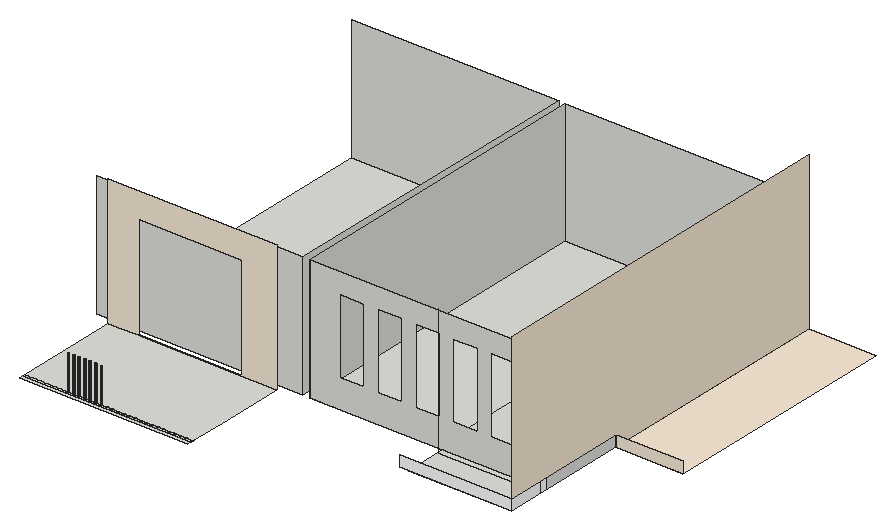
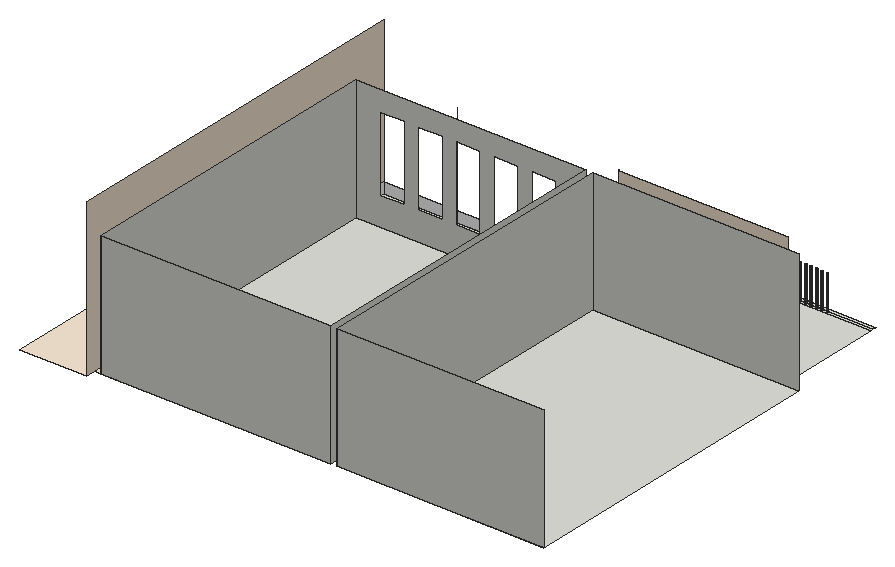
# SketchUp Ruby script. Lengths in inches.
U = 1.inch
M = Sketchup.active_model
def pt(a) = Geom::Point3d.new(a.map { |v| v * U })
def face(e, loops, mat)
  f = e.add_face(loops[0].map { |a| pt(a) })
  loops[1..].each { |l| e.add_face(l.map { |a| pt(a) }).erase! }
  f.material = f.back_material = mat if mat
  f
end
# faces: each face lists its corners as indices into pts; further lists are holes
def faces(e, pts, list, mat = nil) = list.each { |f| face(e, (f[0].is_a?(Array) ? f : [f]).map { |l| l.map { |i| pts[i] } }, mat) }
# xy, xz, yz: faces in a plane at the given z, y or x. An outline is a flat list of corners, or four numbers for a rectangle; further outlines are holes
def ring(l) = l.size == 4 ? [[l[0], l[1]], [l[2], l[1]], [l[2], l[3]], [l[0], l[3]]] : l.each_slice(2).to_a
def flat(e, list, mat, &to3) = list.each { |f| face(e, (f[0].is_a?(Array) ? f : [f]).map { |l| ring(l).map { |u, v| to3.(u, v) } }, mat) }
def xy(e, z, list, mat = nil) = flat(e, list, mat) { |x, y| [x, y, z] }
def xz(e, y, list, mat = nil) = flat(e, list, mat) { |x, z| [x, y, z] }
def yz(e, x, list, mat = nil) = flat(e, list, mat) { |y, z| [x, y, z] }
def lines(e, pts, list) = list.each { |a, b| e.add_line(pt(pts[a]), pt(pts[b])) }
# prism: a flat outline (further loops are holes) pulled along v
def prism(e, loops, v, mat = nil)
  f = face(e, loops, mat); d = Geom::Vector3d.new(v.map { |x| x * U })
  f.pushpull(f.normal.samedirection?(d) ? d.length : -d.length)
end
def box(e, o, s, mat = nil) = prism(e, [[o, [o[0] + s[0], o[1], o[2]], [o[0] + s[0], o[1] + s[1], o[2]], [o[0], o[1] + s[1], o[2]]]], [0, 0, s[2]], mat)
def at(x, y, z, deg = 0) = Geom::Transformation.translation(pt([x, y, z])) * Geom::Transformation.rotation(ORIGIN, Z_AXIS, deg.degrees)
def axes(o, x, y, z) = Geom::Transformation.new([*x, 0, *y, 0, *z, 0, *pt(o).to_a, 1])
def part(name) = M.definitions.add(name)
# library, detail: a bought-in or finely detailed component or shape, given as its bounding box
def library(name, o, s) = part(name).tap { |d| box(d.entities, o, s) }
def detail(e, o, s) = box(e.add_group.entities, o, s)
def put(e, d, t, mat = nil) = e.add_instance(d, t).tap { |i| i.material = mat if mat }
def group(e, t, mat = nil) = e.add_group.tap { |g| g.transformation = t; g.material = mat if mat }.entities
root = M.entities
M.materials.add("[0028_AntiqueWhite]").color = [250, 235, 215]
M.materials.add("[Color M00]").color = [255, 255, 255]
M.materials.add("[Color M08]").color = [30, 30, 30]
xy(root,321,[[206.51,190.32,206.52,193.51,50.75,193.51,50.75,190.5],[206.52,193.51,206.5625,231.9375,206.63,292.44,206.5625,292.44,177.59,292.48,76.05,292.6,50.75,292.625,50.68,231.9375,50.75,231.9375,50.75,196.625,206.52,196.625],[[50.75,193.51,206.52,196.625],[55.99,194.51,55.8,194.57,55.63,194.67,55.5,194.81,55.41,194.99,55.36,195.18,55.37,195.375,55.42,195.5625,55.53,195.73,55.67,195.86,55.84,195.95,56.03,196,56.23,195.99,56.42,195.9375,56.58,195.83,56.72,195.69,56.81,195.52,56.85,195.33,56.85,195.13,56.79,194.95,56.6875,194.78,56.55,194.64,56.375,194.55,56.18,194.51],[61.05,194.51,60.86,194.57,60.7,194.67,60.5625,194.81,60.47,194.99,60.42,195.18,60.43,195.375,60.49,195.5625,60.59,195.73,60.73,195.86,60.9,195.95,61.1,196,61.29,195.99,61.48,195.9375,61.65,195.83,61.78,195.69,61.87,195.52,61.92,195.33,61.91,195.13,61.85,194.95,61.75,194.78,61.61,194.64,61.4375,194.55,61.25,194.51],[66.11,194.51,65.93,194.57,65.76,194.67,65.625,194.81,65.53,194.99,65.49,195.18,65.49,195.375,65.55,195.5625,65.65,195.73,65.79,195.86,65.97,195.95,66.16,196,66.35,195.99,66.54,195.9375,66.71,195.83,66.84,195.69,66.93,195.52,66.98,195.33,66.97,195.13,66.92,194.95,66.8125,194.78,66.67,194.64,66.5,194.55,66.31,194.51],[71.18,194.51,70.99,194.57,70.82,194.67,70.6875,194.81,70.59,194.99,70.55,195.18,70.56,195.375,70.61,195.5625,70.71,195.73,70.86,195.86,71.03,195.95,71.22,196,71.42,195.99,71.6,195.9375,71.77,195.83,71.9,195.69,72,195.52,72.04,195.33,72.04,195.13,71.98,194.95,71.875,194.78,71.73,194.64,71.5625,194.55,71.37,194.51],[76.24,194.51,76.05,194.57,75.88,194.67,75.75,194.81,75.66,194.99,75.61,195.18,75.62,195.375,75.67,195.5625,75.78,195.73,75.92,195.86,76.09,195.95,76.28,196,76.48,195.99,76.67,195.9375,76.83,195.83,76.97,195.69,77.06,195.52,77.1,195.33,77.1,195.13,77.04,194.95,76.9375,194.78,76.8,194.64,76.625,194.55,76.43,194.51],[81.3,194.51,81.11,194.57,80.95,194.67,80.8125,194.81,80.72,194.99,80.67,195.18,80.68,195.375,80.74,195.5625,80.84,195.73,80.98,195.86,81.15,195.95,81.35,196,81.54,195.99,81.73,195.9375,81.9,195.83,82.03,195.69,82.12,195.52,82.17,195.33,82.16,195.13,82.1,194.95,82,194.78,81.86,194.64,81.6875,194.55,81.5,194.51],[86.36,194.51,86.18,194.57,86.01,194.67,85.875,194.81,85.78,194.99,85.74,195.18,85.74,195.375,85.8,195.5625,85.9,195.73,86.04,195.86,86.22,195.95,86.41,196,86.6,195.99,86.79,195.9375,86.96,195.83,87.09,195.69,87.18,195.52,87.23,195.33,87.22,195.13,87.17,194.95,87.0625,194.78,86.92,194.64,86.75,194.55,86.56,194.51],[91.43,194.51,91.24,194.57,91.07,194.67,90.9375,194.81,90.84,194.99,90.8,195.18,90.81,195.375,90.86,195.5625,90.96,195.73,91.11,195.86,91.28,195.95,91.47,196,91.67,195.99,91.85,195.9375,92.02,195.83,92.15,195.69,92.25,195.52,92.29,195.33,92.29,195.13,92.23,194.95,92.125,194.78,91.98,194.64,91.8125,194.55,91.62,194.51],[96.49,194.51,96.3,194.57,96.13,194.67,96,194.81,95.91,194.99,95.86,195.18,95.87,195.375,95.92,195.5625,96.03,195.73,96.17,195.86,96.34,195.95,96.53,196,96.73,195.99,96.92,195.9375,97.08,195.83,97.22,195.69,97.31,195.52,97.35,195.33,97.35,195.13,97.29,194.95,97.1875,194.78,97.05,194.64,96.875,194.55,96.68,194.51],[101.55,194.51,101.36,194.57,101.2,194.67,101.0625,194.81,100.97,194.99,100.92,195.18,100.93,195.375,100.99,195.5625,101.09,195.73,101.23,195.86,101.4,195.95,101.6,196,101.79,195.99,101.98,195.9375,102.15,195.83,102.28,195.69,102.37,195.52,102.42,195.33,102.41,195.13,102.35,194.95,102.25,194.78,102.11,194.64,101.9375,194.55,101.75,194.51],[106.61,194.51,106.43,194.57,106.26,194.67,106.125,194.81,106.03,194.99,105.99,195.18,105.99,195.375,106.05,195.5625,106.15,195.73,106.29,195.86,106.47,195.95,106.66,196,106.85,195.99,107.04,195.9375,107.21,195.83,107.34,195.69,107.43,195.52,107.48,195.33,107.47,195.13,107.42,194.95,107.3125,194.78,107.17,194.64,107,194.55,106.81,194.51],[111.68,194.51,111.49,194.57,111.32,194.67,111.1875,194.81,111.09,194.99,111.05,195.18,111.06,195.375,111.11,195.5625,111.21,195.73,111.36,195.86,111.53,195.95,111.72,196,111.92,195.99,112.1,195.9375,112.27,195.83,112.4,195.69,112.5,195.52,112.54,195.33,112.54,195.13,112.48,194.95,112.375,194.78,112.23,194.64,112.0625,194.55,111.87,194.51],[116.74,194.51,116.55,194.57,116.38,194.67,116.25,194.81,116.16,194.99,116.11,195.18,116.12,195.375,116.17,195.5625,116.28,195.73,116.42,195.86,116.59,195.95,116.78,196,116.98,195.99,117.17,195.9375,117.33,195.83,117.47,195.69,117.56,195.52,117.6,195.33,117.6,195.13,117.54,194.95,117.4375,194.78,117.3,194.64,117.125,194.55,116.93,194.51],[121.8,194.51,121.61,194.57,121.45,194.67,121.3125,194.81,121.22,194.99,121.17,195.18,121.18,195.375,121.24,195.5625,121.34,195.73,121.48,195.86,121.65,195.95,121.85,196,122.04,195.99,122.23,195.9375,122.4,195.83,122.53,195.69,122.62,195.52,122.67,195.33,122.66,195.13,122.6,194.95,122.5,194.78,122.36,194.64,122.1875,194.55,122,194.51],[126.86,194.51,126.68,194.57,126.51,194.67,126.375,194.81,126.28,194.99,126.24,195.18,126.24,195.375,126.3,195.5625,126.4,195.73,126.54,195.86,126.72,195.95,126.91,196,127.1,195.99,127.29,195.9375,127.46,195.83,127.59,195.69,127.68,195.52,127.73,195.33,127.72,195.13,127.67,194.95,127.5625,194.78,127.42,194.64,127.25,194.55,127.06,194.51],[132.11,194.51,131.93,194.57,131.76,194.67,131.625,194.81,131.53,194.99,131.49,195.18,131.49,195.375,131.55,195.5625,131.65,195.73,131.79,195.86,131.97,195.95,132.16,196,132.35,195.99,132.54,195.9375,132.71,195.83,132.84,195.69,132.93,195.52,132.98,195.33,132.97,195.13,132.92,194.95,132.8125,194.78,132.67,194.64,132.5,194.55,132.31,194.51],[137.36,194.51,137.18,194.57,137.01,194.67,136.875,194.81,136.78,194.99,136.74,195.18,136.74,195.375,136.8,195.5625,136.9,195.73,137.04,195.86,137.22,195.95,137.41,196,137.6,195.99,137.79,195.9375,137.96,195.83,138.09,195.69,138.18,195.52,138.23,195.33,138.22,195.13,138.17,194.95,138.0625,194.78,137.92,194.64,137.75,194.55,137.56,194.51],[142.61,194.51,142.43,194.57,142.26,194.67,142.125,194.81,142.03,194.99,141.99,195.18,141.99,195.375,142.05,195.5625,142.15,195.73,142.29,195.86,142.47,195.95,142.66,196,142.85,195.99,143.04,195.9375,143.21,195.83,143.34,195.69,143.43,195.52,143.48,195.33,143.47,195.13,143.42,194.95,143.3125,194.78,143.17,194.64,143,194.55,142.81,194.51],[147.86,194.51,147.68,194.57,147.51,194.67,147.375,194.81,147.28,194.99,147.24,195.18,147.24,195.375,147.3,195.5625,147.4,195.73,147.54,195.86,147.72,195.95,147.91,196,148.1,195.99,148.29,195.9375,148.46,195.83,148.59,195.69,148.68,195.52,148.73,195.33,148.72,195.13,148.67,194.95,148.5625,194.78,148.42,194.64,148.25,194.55,148.06,194.51],[153.11,194.51,152.93,194.57,152.76,194.67,152.625,194.81,152.53,194.99,152.49,195.18,152.49,195.375,152.55,195.5625,152.65,195.73,152.79,195.86,152.97,195.95,153.16,196,153.35,195.99,153.54,195.9375,153.71,195.83,153.84,195.69,153.93,195.52,153.98,195.33,153.97,195.13,153.92,194.95,153.8125,194.78,153.67,194.64,153.5,194.55,153.31,194.51],[158.36,194.51,158.18,194.57,158.01,194.67,157.875,194.81,157.78,194.99,157.74,195.18,157.74,195.375,157.8,195.5625,157.9,195.73,158.04,195.86,158.22,195.95,158.41,196,158.6,195.99,158.79,195.9375,158.96,195.83,159.09,195.69,159.18,195.52,159.23,195.33,159.22,195.13,159.17,194.95,159.0625,194.78,158.92,194.64,158.75,194.55,158.56,194.51],[163.61,194.51,163.43,194.57,163.26,194.67,163.125,194.81,163.03,194.99,162.99,195.18,162.99,195.375,163.05,195.5625,163.15,195.73,163.29,195.86,163.47,195.95,163.66,196,163.85,195.99,164.04,195.9375,164.21,195.83,164.34,195.69,164.43,195.52,164.48,195.33,164.47,195.13,164.42,194.95,164.3125,194.78,164.17,194.64,164,194.55,163.81,194.51],[168.86,194.51,168.68,194.57,168.51,194.67,168.375,194.81,168.28,194.99,168.24,195.18,168.24,195.375,168.3,195.5625,168.4,195.73,168.54,195.86,168.72,195.95,168.91,196,169.1,195.99,169.29,195.9375,169.46,195.83,169.59,195.69,169.68,195.52,169.73,195.33,169.72,195.13,169.67,194.95,169.5625,194.78,169.42,194.64,169.25,194.55,169.06,194.51],[174.11,194.51,173.93,194.57,173.76,194.67,173.625,194.81,173.53,194.99,173.49,195.18,173.49,195.375,173.55,195.5625,173.65,195.73,173.79,195.86,173.97,195.95,174.16,196,174.35,195.99,174.54,195.9375,174.71,195.83,174.84,195.69,174.93,195.52,174.98,195.33,174.97,195.13,174.92,194.95,174.8125,194.78,174.67,194.64,174.5,194.55,174.31,194.51],[179.36,194.51,179.18,194.57,179.01,194.67,178.875,194.81,178.78,194.99,178.74,195.18,178.74,195.375,178.8,195.5625,178.9,195.73,179.04,195.86,179.22,195.95,179.41,196,179.6,195.99,179.79,195.9375,179.96,195.83,180.09,195.69,180.18,195.52,180.23,195.33,180.22,195.13,180.17,194.95,180.0625,194.78,179.92,194.64,179.75,194.55,179.56,194.51],[184.61,194.51,184.43,194.57,184.26,194.67,184.125,194.81,184.03,194.99,183.99,195.18,183.99,195.375,184.05,195.5625,184.15,195.73,184.29,195.86,184.47,195.95,184.66,196,184.85,195.99,185.04,195.9375,185.21,195.83,185.34,195.69,185.43,195.52,185.48,195.33,185.47,195.13,185.42,194.95,185.3125,194.78,185.17,194.64,185,194.55,184.81,194.51],[189.86,194.51,189.68,194.57,189.51,194.67,189.375,194.81,189.28,194.99,189.24,195.18,189.24,195.375,189.3,195.5625,189.4,195.73,189.54,195.86,189.72,195.95,189.91,196,190.1,195.99,190.29,195.9375,190.46,195.83,190.59,195.69,190.68,195.52,190.73,195.33,190.72,195.13,190.67,194.95,190.5625,194.78,190.42,194.64,190.25,194.55,190.06,194.51],[195.11,194.51,194.93,194.57,194.76,194.67,194.625,194.81,194.53,194.99,194.49,195.18,194.49,195.375,194.55,195.5625,194.65,195.73,194.79,195.86,194.97,195.95,195.16,196,195.35,195.99,195.54,195.9375,195.71,195.83,195.84,195.69,195.93,195.52,195.98,195.33,195.97,195.13,195.92,194.95,195.8125,194.78,195.67,194.64,195.5,194.55,195.31,194.51],[200.36,194.51,200.18,194.57,200.01,194.67,199.875,194.81,199.78,194.99,199.74,195.18,199.74,195.375,199.8,195.5625,199.9,195.73,200.04,195.86,200.22,195.95,200.41,196,200.6,195.99,200.79,195.9375,200.96,195.83,201.09,195.69,201.18,195.52,201.23,195.33,201.22,195.13,201.17,194.95,201.0625,194.78,200.92,194.64,200.75,194.55,200.56,194.51],[205.61,194.51,205.43,194.57,205.26,194.67,205.125,194.81,205.03,194.99,204.99,195.18,204.99,195.375,205.05,195.5625,205.15,195.73,205.29,195.86,205.47,195.95,205.66,196,205.85,195.99,206.04,195.9375,206.21,195.83,206.34,195.69,206.43,195.52,206.48,195.33,206.47,195.13,206.42,194.95,206.3125,194.78,206.17,194.64,206,194.55,205.81,194.51]],[355.625,259.125,450.25,292.4375],[355.625,292.4375,450.25,298.4375],
  [35.1875,298.4375,226.3125,592.9375],[232.3125,298.4375,349.625,592.9375],[349.625,298.4375,444.4375,592.9375],[444.4375,298.4375,450.25,379.25],[444.4375,379.25,450.25,384.87]])
xy(root,321,[[450.25,379.25,512.4375,601.9375],[444.4375,384.87,450.25,592.9375]],"[0028_AntiqueWhite]")
xy(root,321,[[91.43,194.51,91.24,194.57,91.07,194.67,90.9375,194.81,90.84,194.99,90.8,195.18,90.81,195.375,90.86,195.5625,90.96,195.73,91.11,195.86,91.28,195.95,91.47,196,91.67,195.99,91.85,195.9375,92.02,195.83,92.15,195.69,92.25,195.52,92.29,195.33,92.29,195.13,92.23,194.95,92.125,194.78,91.98,194.64,91.8125,194.55,91.62,194.51],[96.49,194.51,96.3,194.57,96.13,194.67,96,194.81,95.91,194.99,95.86,195.18,95.87,195.375,95.92,195.5625,96.03,195.73,96.17,195.86,96.34,195.95,96.53,196,96.73,195.99,96.92,195.9375,97.08,195.83,97.22,195.69,97.31,195.52,97.35,195.33,97.35,195.13,97.29,194.95,97.1875,194.78,97.05,194.64,96.875,194.55,96.68,194.51],[101.55,194.51,101.36,194.57,101.2,194.67,101.0625,194.81,100.97,194.99,100.92,195.18,100.93,195.375,100.99,195.5625,101.09,195.73,101.23,195.86,101.4,195.95,101.6,196,101.79,195.99,101.98,195.9375,102.15,195.83,102.28,195.69,102.37,195.52,102.42,195.33,102.41,195.13,102.35,194.95,102.25,194.78,102.11,194.64,101.9375,194.55,101.75,194.51],[106.61,194.51,106.43,194.57,106.26,194.67,106.125,194.81,106.03,194.99,105.99,195.18,105.99,195.375,106.05,195.5625,106.15,195.73,106.29,195.86,106.47,195.95,106.66,196,106.85,195.99,107.04,195.9375,107.21,195.83,107.34,195.69,107.43,195.52,107.48,195.33,107.47,195.13,107.42,194.95,107.3125,194.78,107.17,194.64,107,194.55,106.81,194.51],[111.68,194.51,111.49,194.57,111.32,194.67,111.1875,194.81,111.09,194.99,111.05,195.18,111.06,195.375,111.11,195.5625,111.21,195.73,111.36,195.86,111.53,195.95,111.72,196,111.92,195.99,112.1,195.9375,112.27,195.83,112.4,195.69,112.5,195.52,112.54,195.33,112.54,195.13,112.48,194.95,112.375,194.78,112.23,194.64,112.0625,194.55,111.87,194.51],
  [116.74,194.51,116.55,194.57,116.38,194.67,116.25,194.81,116.16,194.99,116.11,195.18,116.12,195.375,116.17,195.5625,116.28,195.73,116.42,195.86,116.59,195.95,116.78,196,116.98,195.99,117.17,195.9375,117.33,195.83,117.47,195.69,117.56,195.52,117.6,195.33,117.6,195.13,117.54,194.95,117.4375,194.78,117.3,194.64,117.125,194.55,116.93,194.51],[121.8,194.51,121.61,194.57,121.45,194.67,121.3125,194.81,121.22,194.99,121.17,195.18,121.18,195.375,121.24,195.5625,121.34,195.73,121.48,195.86,121.65,195.95,121.85,196,122.04,195.99,122.23,195.9375,122.4,195.83,122.53,195.69,122.62,195.52,122.67,195.33,122.66,195.13,122.6,194.95,122.5,194.78,122.36,194.64,122.1875,194.55,122,194.51],[126.86,194.51,126.68,194.57,126.51,194.67,126.375,194.81,126.28,194.99,126.24,195.18,126.24,195.375,126.3,195.5625,126.4,195.73,126.54,195.86,126.72,195.95,126.91,196,127.1,195.99,127.29,195.9375,127.46,195.83,127.59,195.69,127.68,195.52,127.73,195.33,127.72,195.13,127.67,194.95,127.5625,194.78,127.42,194.64,127.25,194.55,127.06,194.51],[132.11,194.51,131.93,194.57,131.76,194.67,131.625,194.81,131.53,194.99,131.49,195.18,131.49,195.375,131.55,195.5625,131.65,195.73,131.79,195.86,131.97,195.95,132.16,196,132.35,195.99,132.54,195.9375,132.71,195.83,132.84,195.69,132.93,195.52,132.98,195.33,132.97,195.13,132.92,194.95,132.8125,194.78,132.67,194.64,132.5,194.55,132.31,194.51],[137.36,194.51,137.18,194.57,137.01,194.67,136.875,194.81,136.78,194.99,136.74,195.18,136.74,195.375,136.8,195.5625,136.9,195.73,137.04,195.86,137.22,195.95,137.41,196,137.6,195.99,137.79,195.9375,137.96,195.83,138.09,195.69,138.18,195.52,138.23,195.33,138.22,195.13,138.17,194.95,138.0625,194.78,137.92,194.64,137.75,194.55,137.56,194.51],
  [142.61,194.51,142.43,194.57,142.26,194.67,142.125,194.81,142.03,194.99,141.99,195.18,141.99,195.375,142.05,195.5625,142.15,195.73,142.29,195.86,142.47,195.95,142.66,196,142.85,195.99,143.04,195.9375,143.21,195.83,143.34,195.69,143.43,195.52,143.48,195.33,143.47,195.13,143.42,194.95,143.3125,194.78,143.17,194.64,143,194.55,142.81,194.51],[147.86,194.51,147.68,194.57,147.51,194.67,147.375,194.81,147.28,194.99,147.24,195.18,147.24,195.375,147.3,195.5625,147.4,195.73,147.54,195.86,147.72,195.95,147.91,196,148.1,195.99,148.29,195.9375,148.46,195.83,148.59,195.69,148.68,195.52,148.73,195.33,148.72,195.13,148.67,194.95,148.5625,194.78,148.42,194.64,148.25,194.55,148.06,194.51],[153.11,194.51,152.93,194.57,152.76,194.67,152.625,194.81,152.53,194.99,152.49,195.18,152.49,195.375,152.55,195.5625,152.65,195.73,152.79,195.86,152.97,195.95,153.16,196,153.35,195.99,153.54,195.9375,153.71,195.83,153.84,195.69,153.93,195.52,153.98,195.33,153.97,195.13,153.92,194.95,153.8125,194.78,153.67,194.64,153.5,194.55,153.31,194.51],[158.36,194.51,158.18,194.57,158.01,194.67,157.875,194.81,157.78,194.99,157.74,195.18,157.74,195.375,157.8,195.5625,157.9,195.73,158.04,195.86,158.22,195.95,158.41,196,158.6,195.99,158.79,195.9375,158.96,195.83,159.09,195.69,159.18,195.52,159.23,195.33,159.22,195.13,159.17,194.95,159.0625,194.78,158.92,194.64,158.75,194.55,158.56,194.51],[163.61,194.51,163.43,194.57,163.26,194.67,163.125,194.81,163.03,194.99,162.99,195.18,162.99,195.375,163.05,195.5625,163.15,195.73,163.29,195.86,163.47,195.95,163.66,196,163.85,195.99,164.04,195.9375,164.21,195.83,164.34,195.69,164.43,195.52,164.48,195.33,164.47,195.13,164.42,194.95,164.3125,194.78,164.17,194.64,164,194.55,163.81,194.51],
  [168.86,194.51,168.68,194.57,168.51,194.67,168.375,194.81,168.28,194.99,168.24,195.18,168.24,195.375,168.3,195.5625,168.4,195.73,168.54,195.86,168.72,195.95,168.91,196,169.1,195.99,169.29,195.9375,169.46,195.83,169.59,195.69,169.68,195.52,169.73,195.33,169.72,195.13,169.67,194.95,169.5625,194.78,169.42,194.64,169.25,194.55,169.06,194.51],[174.11,194.51,173.93,194.57,173.76,194.67,173.625,194.81,173.53,194.99,173.49,195.18,173.49,195.375,173.55,195.5625,173.65,195.73,173.79,195.86,173.97,195.95,174.16,196,174.35,195.99,174.54,195.9375,174.71,195.83,174.84,195.69,174.93,195.52,174.98,195.33,174.97,195.13,174.92,194.95,174.8125,194.78,174.67,194.64,174.5,194.55,174.31,194.51],[179.36,194.51,179.18,194.57,179.01,194.67,178.875,194.81,178.78,194.99,178.74,195.18,178.74,195.375,178.8,195.5625,178.9,195.73,179.04,195.86,179.22,195.95,179.41,196,179.6,195.99,179.79,195.9375,179.96,195.83,180.09,195.69,180.18,195.52,180.23,195.33,180.22,195.13,180.17,194.95,180.0625,194.78,179.92,194.64,179.75,194.55,179.56,194.51],[184.61,194.51,184.43,194.57,184.26,194.67,184.125,194.81,184.03,194.99,183.99,195.18,183.99,195.375,184.05,195.5625,184.15,195.73,184.29,195.86,184.47,195.95,184.66,196,184.85,195.99,185.04,195.9375,185.21,195.83,185.34,195.69,185.43,195.52,185.48,195.33,185.47,195.13,185.42,194.95,185.3125,194.78,185.17,194.64,185,194.55,184.81,194.51],[189.86,194.51,189.68,194.57,189.51,194.67,189.375,194.81,189.28,194.99,189.24,195.18,189.24,195.375,189.3,195.5625,189.4,195.73,189.54,195.86,189.72,195.95,189.91,196,190.1,195.99,190.29,195.9375,190.46,195.83,190.59,195.69,190.68,195.52,190.73,195.33,190.72,195.13,190.67,194.95,190.5625,194.78,190.42,194.64,190.25,194.55,190.06,194.51],
  [195.11,194.51,194.93,194.57,194.76,194.67,194.625,194.81,194.53,194.99,194.49,195.18,194.49,195.375,194.55,195.5625,194.65,195.73,194.79,195.86,194.97,195.95,195.16,196,195.35,195.99,195.54,195.9375,195.71,195.83,195.84,195.69,195.93,195.52,195.98,195.33,195.97,195.13,195.92,194.95,195.8125,194.78,195.67,194.64,195.5,194.55,195.31,194.51],[200.36,194.51,200.18,194.57,200.01,194.67,199.875,194.81,199.78,194.99,199.74,195.18,199.74,195.375,199.8,195.5625,199.9,195.73,200.04,195.86,200.22,195.95,200.41,196,200.6,195.99,200.79,195.9375,200.96,195.83,201.09,195.69,201.18,195.52,201.23,195.33,201.22,195.13,201.17,194.95,201.0625,194.78,200.92,194.64,200.75,194.55,200.56,194.51],[205.61,194.51,205.43,194.57,205.26,194.67,205.125,194.81,205.03,194.99,204.99,195.18,204.99,195.375,205.05,195.5625,205.15,195.73,205.29,195.86,205.47,195.95,205.66,196,205.85,195.99,206.04,195.9375,206.21,195.83,206.34,195.69,206.43,195.52,206.48,195.33,206.47,195.13,206.42,194.95,206.3125,194.78,206.17,194.64,206,194.55,205.81,194.51]],"[Color M08]")
xz(root,194.51,[[91.43,321,91.62,353.72],[96.49,321,96.68,353.72],[101.55,321,101.75,353.72],[106.61,321,106.81,353.72],[111.68,321,111.87,353.72],
  [116.74,321,116.93,353.72]],"[Color M08]")
xz(root,259.125,[[346.5625,321,450.25,331.3125]],"[Color M00]")
xz(root,298.4375,[[35.1875,321,226.3125,435],[[232.3125,321,444.4375,435],[329.81,347.02,352.43,416.46],[364.87,347.02,387.5,416.46],[399.93,347.02,422.56,416.46],[294.75,347.02,317.37,416.46],[259.68,347.02,282.31,416.46]]])
xz(root,379.25,[[450.25,321,512.4375,331.3125]],"[0028_AntiqueWhite]")
xz(root,592.9375,[[35.1875,321,226.3125,435],[232.3125,321,444.4375,435]])
yz(root,92.29,[[195.13,321,195.33,353.72]],"[Color M08]")
yz(root,97.35,[[195.13,321,195.33,353.72]],"[Color M08]")
yz(root,105.99,[[195.18,321,195.375,353.72]],"[Color M08]")
yz(root,112.54,[[195.13,321,195.33,353.72]],"[Color M08]")
yz(root,117.6,[[195.13,321,195.33,353.72]],"[Color M08]")
yz(root,226.3125,[[298.4375,321,592.9375,435]])
yz(root,232.3125,[[298.4375,321,592.9375,435]])
yz(root,444.4375,[[298.4375,321,592.9375,435]])
yz(root,450.25,[[298.4375,321,379.25,331.3125]])
yz(root,450.25,[[379.25,321,601.9375,321,601.9375,465,259.125,465,259.125,331.3125,379.25,331.3125]],"[0028_AntiqueWhite]")
yz(root,450.25,[[259.125,321,292.4375,331.3125],[292.4375,321,298.4375,331.3125]],"[Color M00]")
p = [[91.62,194.51,321],[91.8125,194.55,321],[91.8125,194.55,353.72],[91.62,194.51,353.72],[96.3,194.57,321],[96.49,194.51,321],
  [96.49,194.51,353.72],[96.3,194.57,353.72],[96.68,194.51,321],[96.875,194.55,321],[96.875,194.55,353.72],[96.68,194.51,353.72],
  [101.36,194.57,321],[101.55,194.51,321],[101.55,194.51,353.72],[101.36,194.57,353.72],[101.75,194.51,321],[101.9375,194.55,321],
  [101.9375,194.55,353.72],[101.75,194.51,353.72],[106.43,194.57,321],[106.61,194.51,321],[106.61,194.51,353.72],[106.43,194.57,353.72],
  [106.81,194.51,321],[107,194.55,321],[107,194.55,353.72],[106.81,194.51,353.72],[111.49,194.57,321],[111.68,194.51,321],
  [111.68,194.51,353.72],[111.49,194.57,353.72],[111.87,194.51,321],[112.0625,194.55,321],[112.0625,194.55,353.72],[111.87,194.51,353.72],
  [116.55,194.57,321],[116.74,194.51,321],[116.74,194.51,353.72],[116.55,194.57,353.72],[116.93,194.51,321],[117.125,194.55,321],
  [117.125,194.55,353.72],[116.93,194.51,353.72],[91.98,194.64,321],[91.98,194.64,353.72],[92.125,194.78,321],[92.125,194.78,353.72],
  [96.13,194.67,321],[96.13,194.67,353.72],[97.05,194.64,321],[97.05,194.64,353.72],[97.1875,194.78,321],[97.1875,194.78,353.72],
  [101.2,194.67,321],[101.2,194.67,353.72],[102.11,194.64,321],[102.11,194.64,353.72],[102.25,194.78,321],[102.25,194.78,353.72],
  [106.26,194.67,321],[106.26,194.67,353.72],[107.17,194.64,321],[107.17,194.64,353.72],[107.3125,194.78,321],[107.3125,194.78,353.72],
  [111.32,194.67,321],[111.32,194.67,353.72],[112.23,194.64,321],[112.23,194.64,353.72],[112.375,194.78,321],[112.375,194.78,353.72],
  [116.38,194.67,321],[116.38,194.67,353.72],[117.3,194.64,321],[117.3,194.64,353.72],[117.4375,194.78,321],[117.4375,194.78,353.72],
  [122.36,194.64,321],[122.5,194.78,321],[122.5,194.78,353.72],[122.36,194.64,353.72],[96,194.81,321],[96,194.81,353.72],
  [101.0625,194.81,321],[101.0625,194.81,353.72],[106.125,194.81,321],[106.125,194.81,353.72],[111.1875,194.81,321],[111.1875,194.81,353.72],
  [116.25,194.81,321],[116.25,194.81,353.72],[92.23,194.95,321],[92.23,194.95,353.72],[95.91,194.99,321],[95.91,194.99,353.72],
  [97.29,194.95,321],[97.29,194.95,353.72],[100.97,194.99,321],[100.97,194.99,353.72],[102.35,194.95,321],[102.35,194.95,353.72],
  [106.03,194.99,321],[106.03,194.99,353.72],[107.42,194.95,321],[107.42,194.95,353.72],[111.09,194.99,321],[111.09,194.99,353.72],
  [112.48,194.95,321],[112.48,194.95,353.72],[116.16,194.99,321],[116.16,194.99,353.72],[117.54,194.95,321],[117.54,194.95,353.72],
  [122.6,194.95,321],[122.6,194.95,353.72],[92.29,195.13,321],[92.29,195.13,353.72],[97.35,195.13,321],[97.35,195.13,353.72],
  [102.41,195.13,321],[102.41,195.13,353.72],[107.47,195.13,321],[107.47,195.13,353.72],[112.54,195.13,321],[112.54,195.13,353.72],
  [117.6,195.13,321],[117.6,195.13,353.72],[122.66,195.13,321],[122.66,195.13,353.72],[95.86,195.18,321],[95.86,195.18,353.72],
  [100.92,195.18,321],[100.92,195.18,353.72],[105.99,195.18,321],[105.99,195.18,353.72],[111.05,195.18,321],[111.05,195.18,353.72],
  [116.11,195.18,321],[116.11,195.18,353.72],[102.42,195.33,321],[102.42,195.33,353.72],[107.48,195.33,321],[107.48,195.33,353.72],
  [122.67,195.33,321],[122.67,195.33,353.72],[95.87,195.375,321],[95.87,195.375,353.72],[100.93,195.375,321],[100.93,195.375,353.72],
  [111.06,195.375,321],[111.06,195.375,353.72],[116.12,195.375,321],[116.12,195.375,353.72],[92.29,195.33,321],[92.25,195.52,321],
  [92.25,195.52,353.72],[92.29,195.33,353.72],[97.35,195.33,321],[97.31,195.52,321],[97.31,195.52,353.72],[97.35,195.33,353.72],
  [102.37,195.52,321],[102.37,195.52,353.72],[107.43,195.52,321],[107.43,195.52,353.72],[112.54,195.33,321],[112.5,195.52,321],
  [112.5,195.52,353.72],[112.54,195.33,353.72],[117.6,195.33,321],[117.56,195.52,321],[117.56,195.52,353.72],[117.6,195.33,353.72],
  [122.62,195.52,321],[122.62,195.52,353.72],[95.92,195.5625,321],[95.92,195.5625,353.72],[100.99,195.5625,321],[100.99,195.5625,353.72],
  [106.05,195.5625,321],[105.99,195.375,321],[105.99,195.375,353.72],[106.05,195.5625,353.72],[111.11,195.5625,321],[111.11,195.5625,353.72],
  [116.17,195.5625,321],[116.17,195.5625,353.72],[92.15,195.69,321],[92.15,195.69,353.72],[97.22,195.69,321],[97.22,195.69,353.72],
  [102.28,195.69,321],[102.28,195.69,353.72],[107.34,195.69,321],[107.34,195.69,353.72],[112.4,195.69,321],[112.4,195.69,353.72],
  [117.47,195.69,321],[117.47,195.69,353.72],[122.53,195.69,321],[122.53,195.69,353.72],[96.03,195.73,321],[96.03,195.73,353.72],
  [101.09,195.73,321],[101.09,195.73,353.72],[106.15,195.73,321],[106.15,195.73,353.72],[111.21,195.73,321],[111.21,195.73,353.72],
  [116.28,195.73,321],[116.28,195.73,353.72],[92.02,195.83,321],[92.02,195.83,353.72],[96.17,195.86,321],[96.17,195.86,353.72],
  [97.08,195.83,321],[97.08,195.83,353.72],[101.23,195.86,321],[101.23,195.86,353.72],[102.15,195.83,321],[102.15,195.83,353.72],
  [106.29,195.86,321],[106.29,195.86,353.72],[107.21,195.83,321],[107.21,195.83,353.72],[111.36,195.86,321],[111.36,195.86,353.72],
  [112.27,195.83,321],[112.27,195.83,353.72],[116.42,195.86,321],[116.42,195.86,353.72],[117.33,195.83,321],[117.33,195.83,353.72],
  [91.85,195.9375,321],[91.85,195.9375,353.72],[96.92,195.9375,321],[96.92,195.9375,353.72],[101.98,195.9375,321],[101.98,195.9375,353.72],
  [107.04,195.9375,321],[107.04,195.9375,353.72],[112.1,195.9375,321],[112.1,195.9375,353.72],[117.17,195.9375,321],[117.17,195.9375,353.72],
  [91.67,195.99,321],[91.67,195.99,353.72],[96.34,195.95,321],[96.34,195.95,353.72],[96.73,195.99,321],[96.73,195.99,353.72],
  [101.4,195.95,321],[101.4,195.95,353.72],[101.79,195.99,321],[101.79,195.99,353.72],[106.47,195.95,321],[106.47,195.95,353.72],
  [106.85,195.99,321],[106.85,195.99,353.72],[111.53,195.95,321],[111.53,195.95,353.72],[111.92,195.99,321],[111.92,195.99,353.72],
  [116.59,195.95,321],[116.59,195.95,353.72],[116.98,195.99,321],[116.98,195.99,353.72],[91.47,196,321],[91.28,195.95,321],
  [91.28,195.95,353.72],[91.47,196,353.72],[96.53,196,321],[96.53,196,353.72],[101.6,196,321],[101.6,196,353.72],
  [106.66,196,321],[106.66,196,353.72],[111.72,196,321],[111.72,196,353.72],[116.78,196,321],[116.78,196,353.72],
  [50.75,292.625,321],[76.05,292.6,321],[177.59,292.48,321],[206.5625,292.44,321],[206.5625,292.44,441],[206.3125,292.44,441],
  [50.75,292.625,441],[50.75,292.625,321.02],[174.56,292.48,417.3125],[174.56,292.48,321.4375],[78.68,292.59,321.4375],[78.68,292.59,417.3125],
  [355.625,292.4375,321],[355.625,292.4375,441]]
faces(root,p,[[0,1,2,3],[4,5,6,7],[8,9,10,11],[12,13,14,15],[16,17,18,19],[20,21,22,23],[24,25,26,27],[28,29,30,31],
  [32,33,34,35],[36,37,38,39],[40,41,42,43],[1,44,45,2],[44,46,47,45],[48,4,7,49],[9,50,51,10],[50,52,53,51],
  [54,12,15,55],[17,56,57,18],[56,58,59,57],[60,20,23,61],[25,62,63,26],[62,64,65,63],[66,28,31,67],[33,68,69,34],
  [68,70,71,69],[72,36,39,73],[41,74,75,42],[74,76,77,75],[78,79,80,81],[82,48,49,83],[84,54,55,85],[86,60,61,87],
  [88,66,67,89],[90,72,73,91],[46,92,93,47],[94,82,83,95],[52,96,97,53],[98,84,85,99],[58,100,101,59],[102,86,87,103],
  [64,104,105,65],[106,88,89,107],[70,108,109,71],[110,90,91,111],[76,112,113,77],[79,114,115,80],[92,116,117,93],[96,118,119,97],
  [100,120,121,101],[104,122,123,105],[108,124,125,109],[112,126,127,113],[114,128,129,115],[130,94,95,131],[132,98,99,133],[134,102,103,135],
  [136,106,107,137],[138,110,111,139],[120,140,141,121],[122,142,143,123],[128,144,145,129],[146,130,131,147],[148,132,133,149],[150,136,137,151],
  [152,138,139,153],[154,155,156,157],[158,159,160,161],[140,162,163,141],[142,164,165,143],[166,167,168,169],[170,171,172,173],[144,174,175,145],
  [176,146,147,177],[178,148,149,179],[180,181,182,183],[184,150,151,185],[186,152,153,187],[155,188,189,156],[159,190,191,160],[162,192,193,163],
  [164,194,195,165],[167,196,197,168],[171,198,199,172],[174,200,201,175],[202,176,177,203],[204,178,179,205],[206,180,183,207],[208,184,185,209],
  [210,186,187,211],[188,212,213,189],[214,202,203,215],[190,216,217,191],[218,204,205,219],[192,220,221,193],[222,206,207,223],[194,224,225,195],
  [226,208,209,227],[196,228,229,197],[230,210,211,231],[198,232,233,199],[212,234,235,213],[216,236,237,217],[220,238,239,221],[224,240,241,225],
  [228,242,243,229],[232,244,245,233],[234,246,247,235],[248,214,215,249],[236,250,251,237],[252,218,219,253],[238,254,255,239],[256,222,223,257],
  [240,258,259,241],[260,226,227,261],[242,262,263,243],[264,230,231,265],[244,266,267,245],[268,269,270,271],[246,268,271,247],[272,248,249,273],
  [250,272,273,251],[274,252,253,275],[254,274,275,255],[276,256,257,277],[258,276,277,259],[278,260,261,279],[262,278,279,263],[280,264,265,281],
  [266,280,281,267]],"[Color M08]")
faces(root,p,[[[282,283,284,285,286,287,288,289],[290,291,292,293]]],"[0028_AntiqueWhite]")
lines(root,p,[[294,295]])
